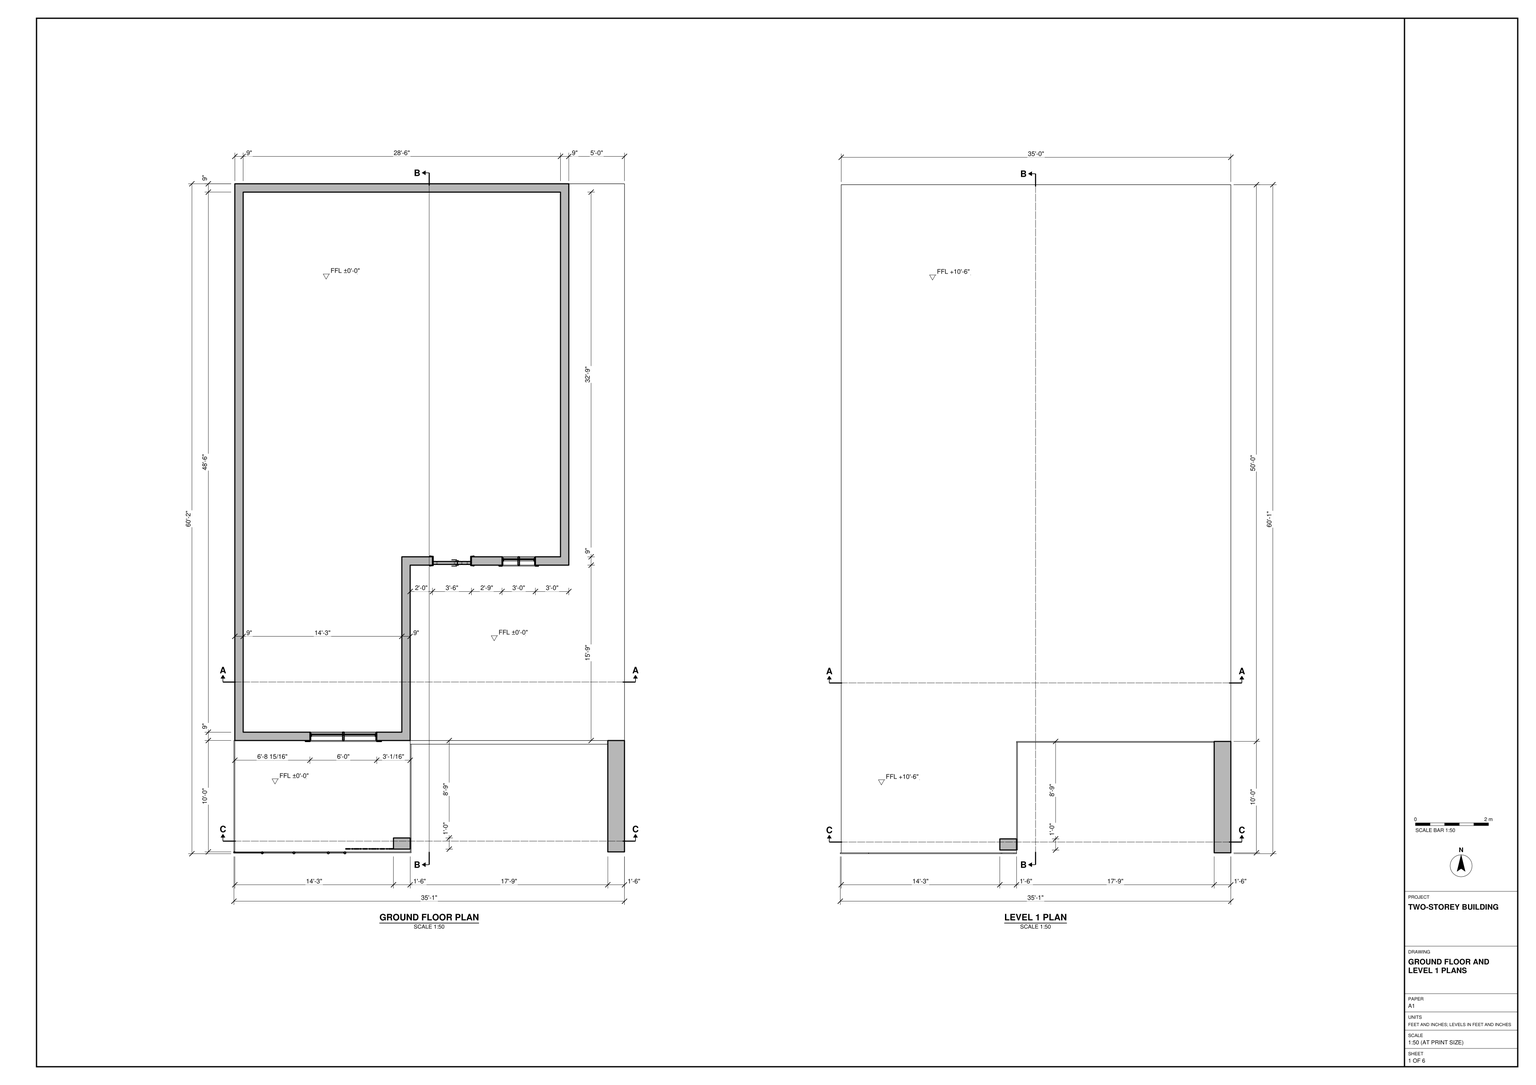
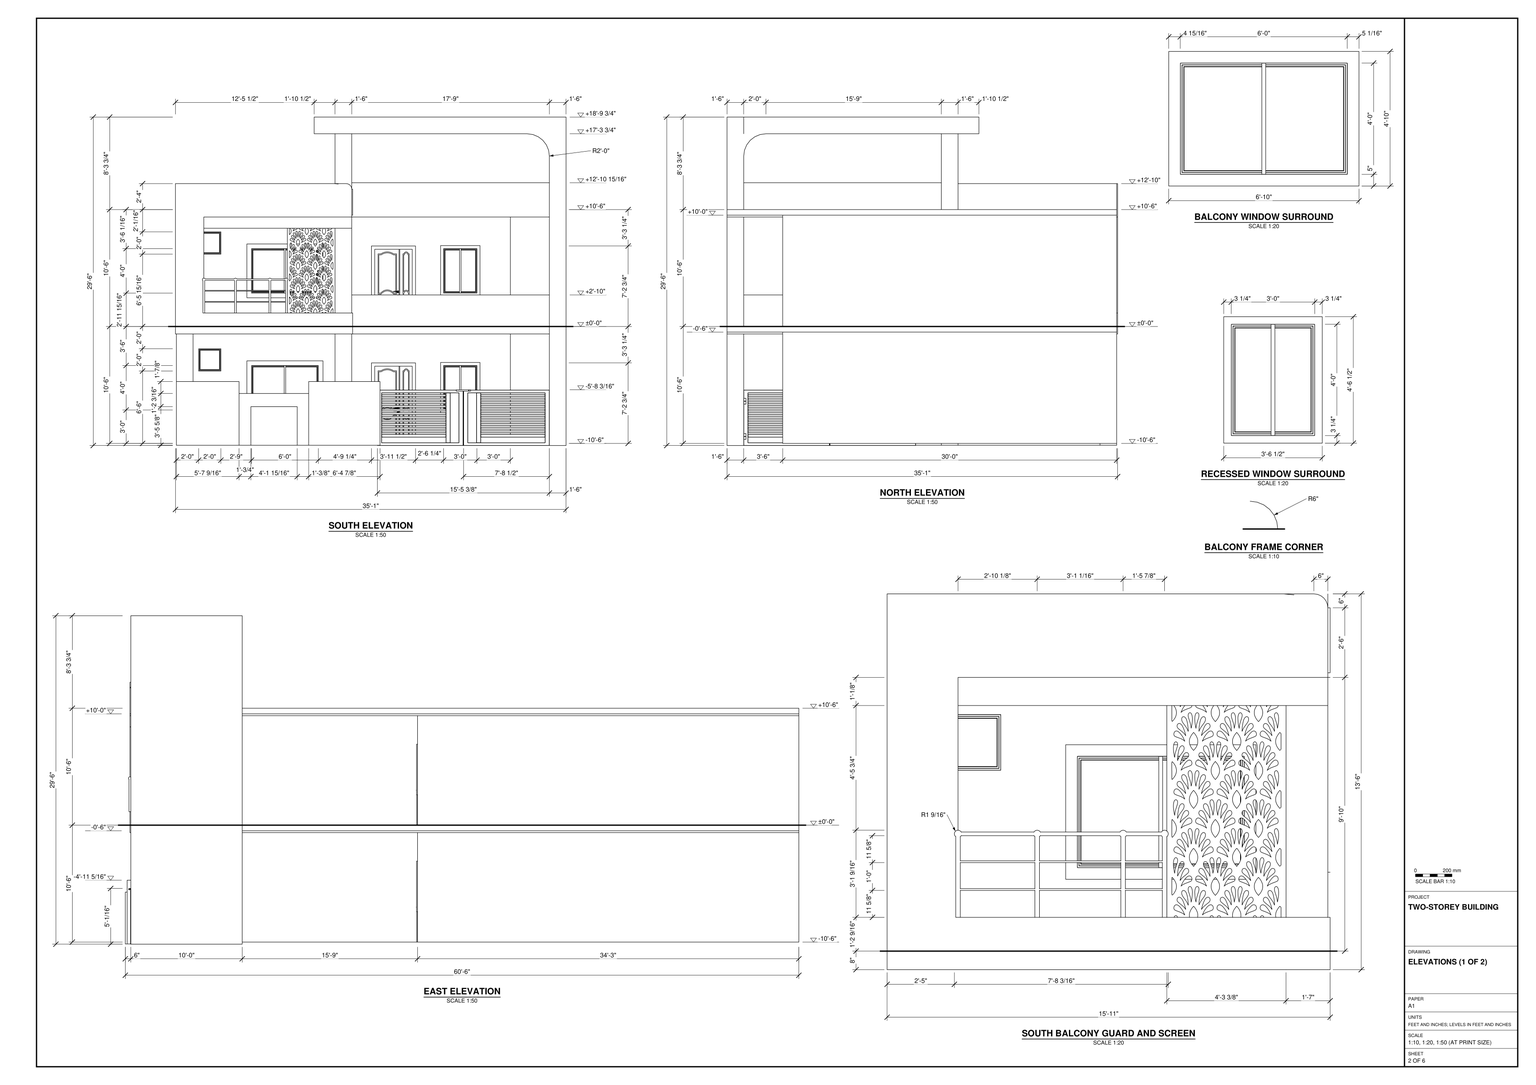
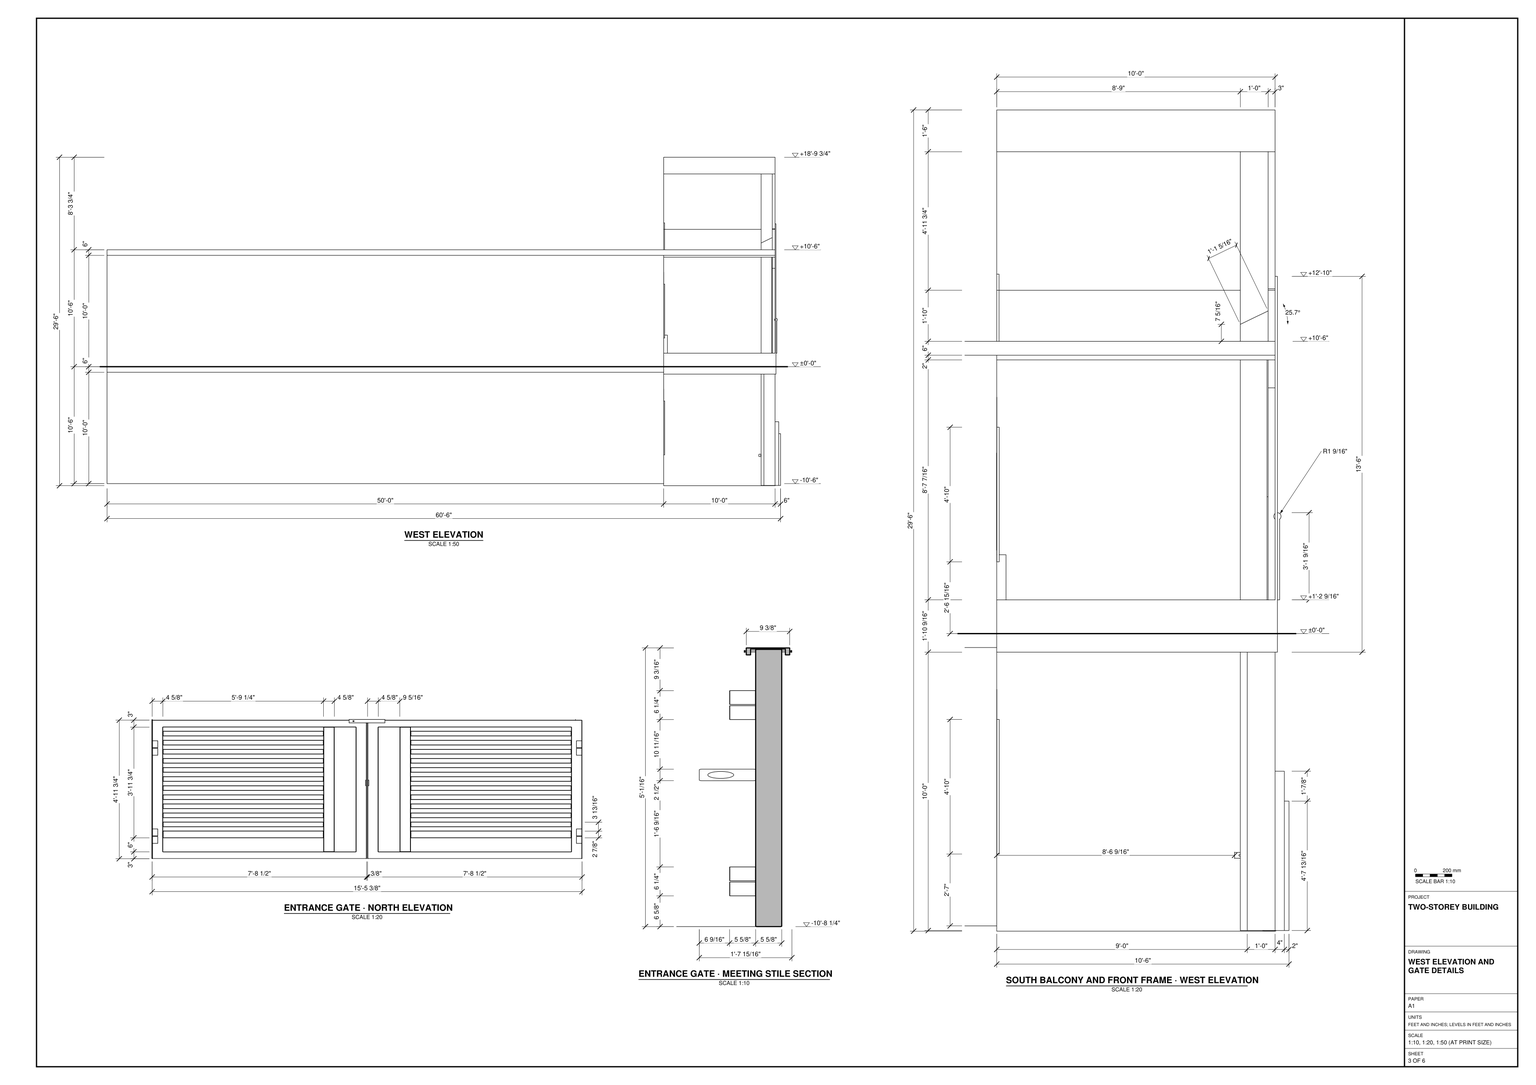
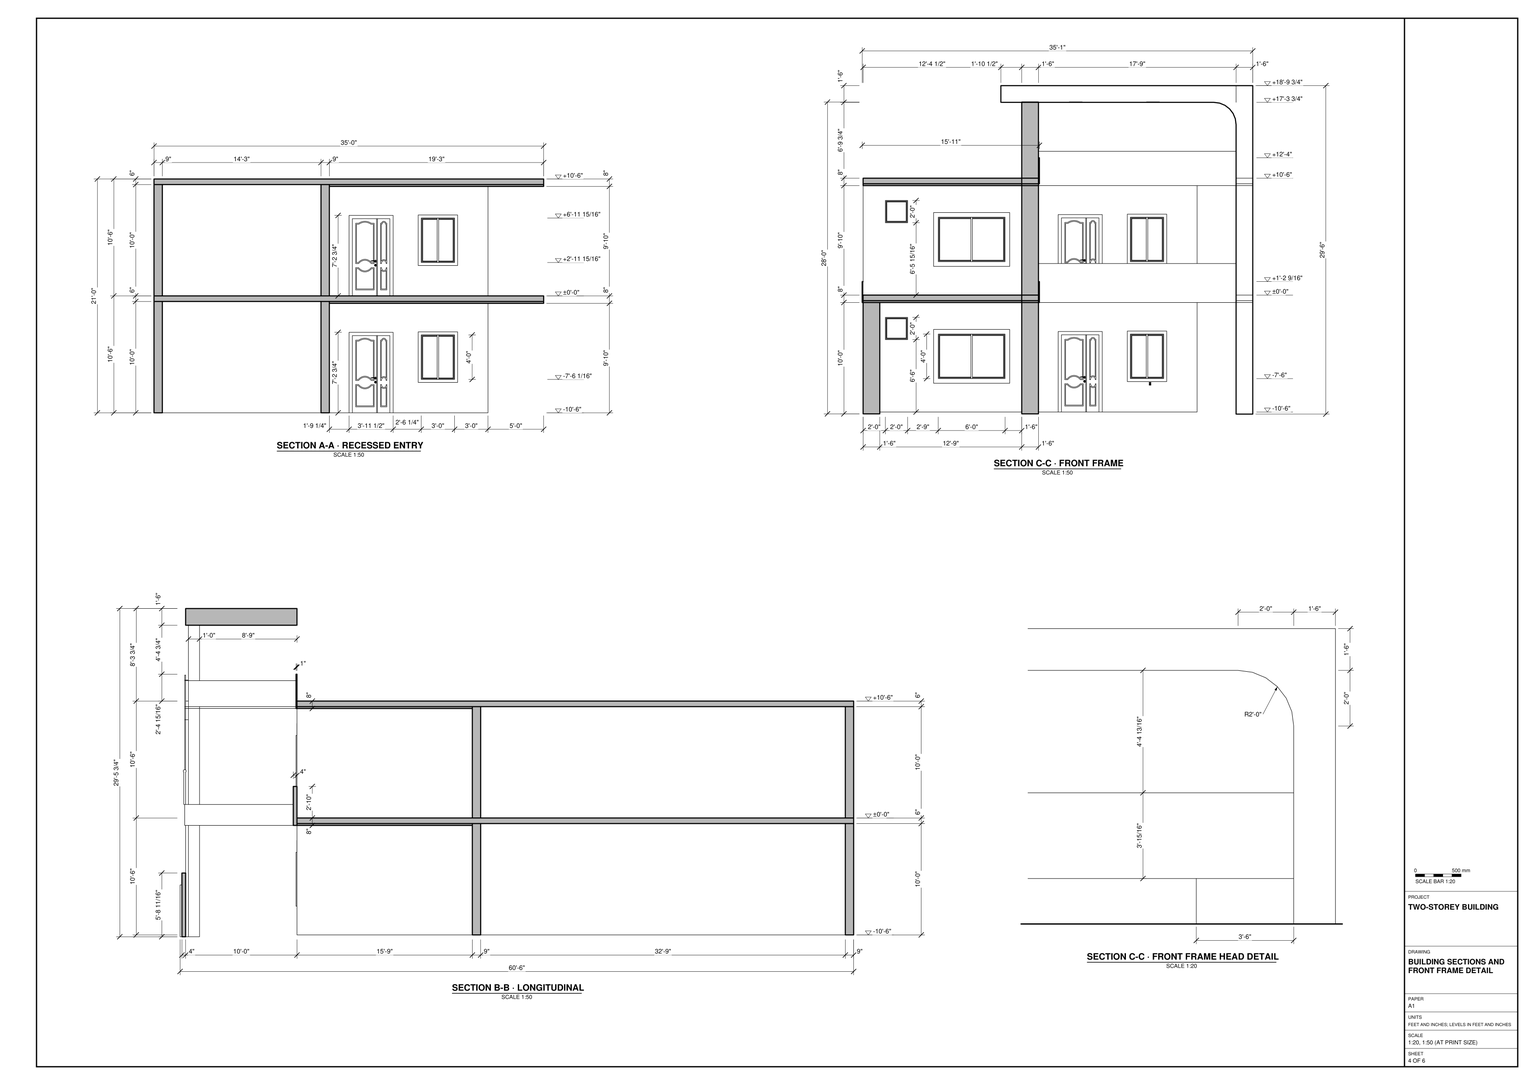
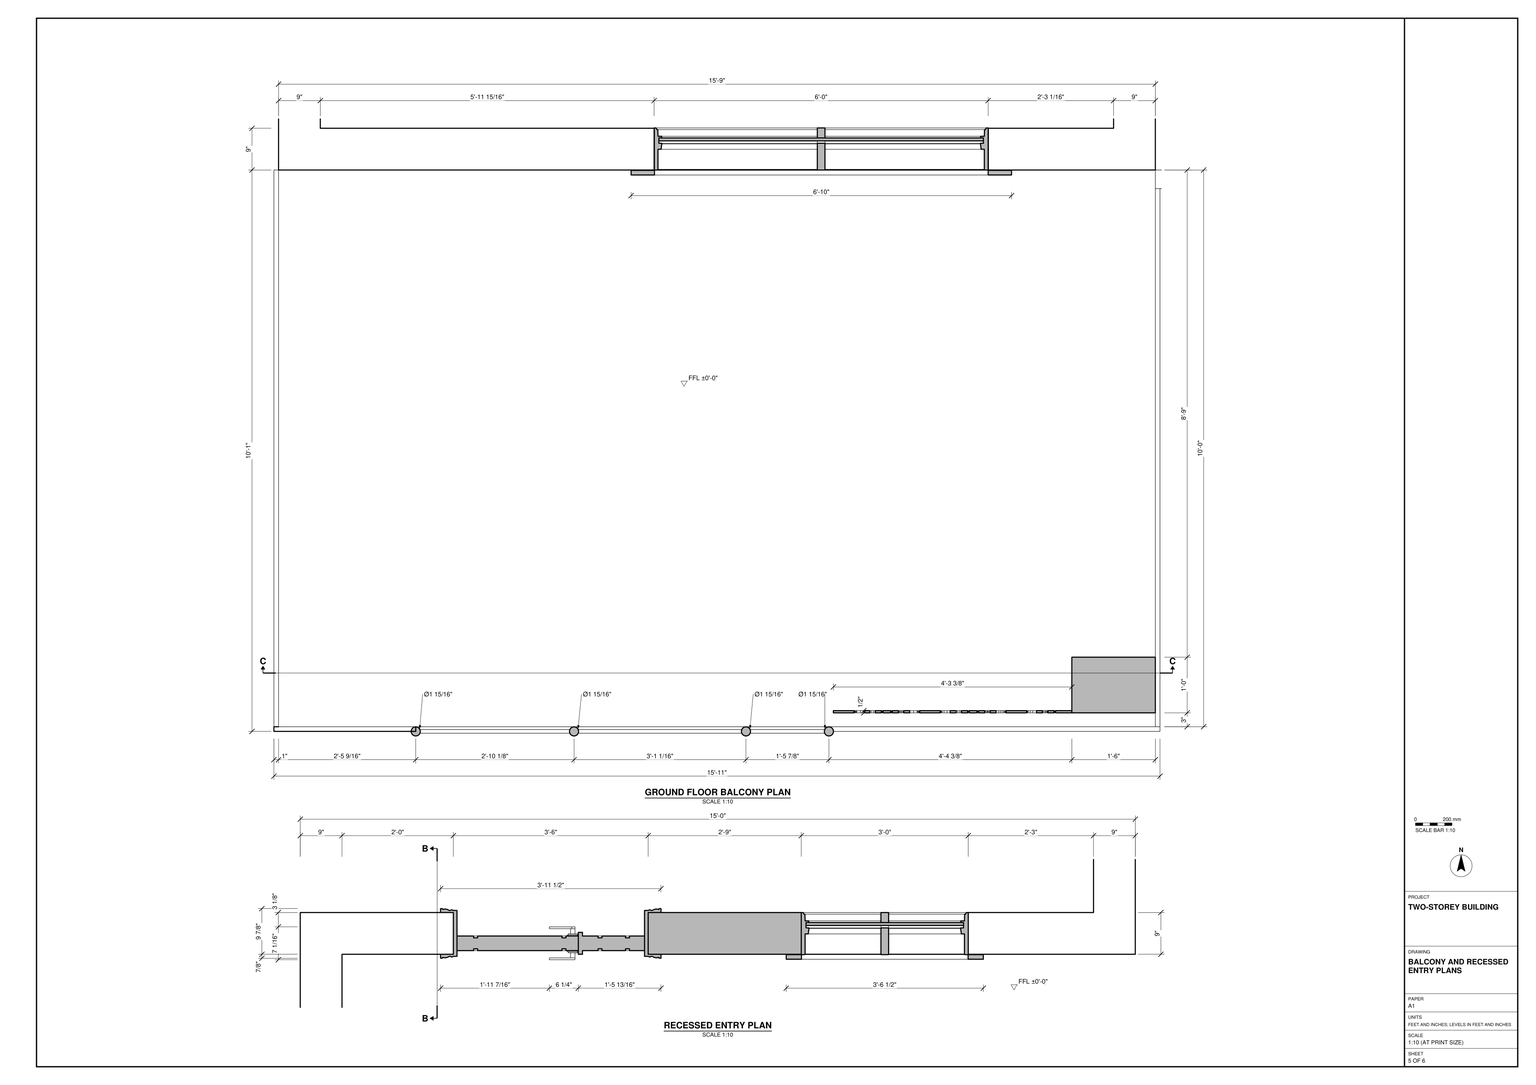
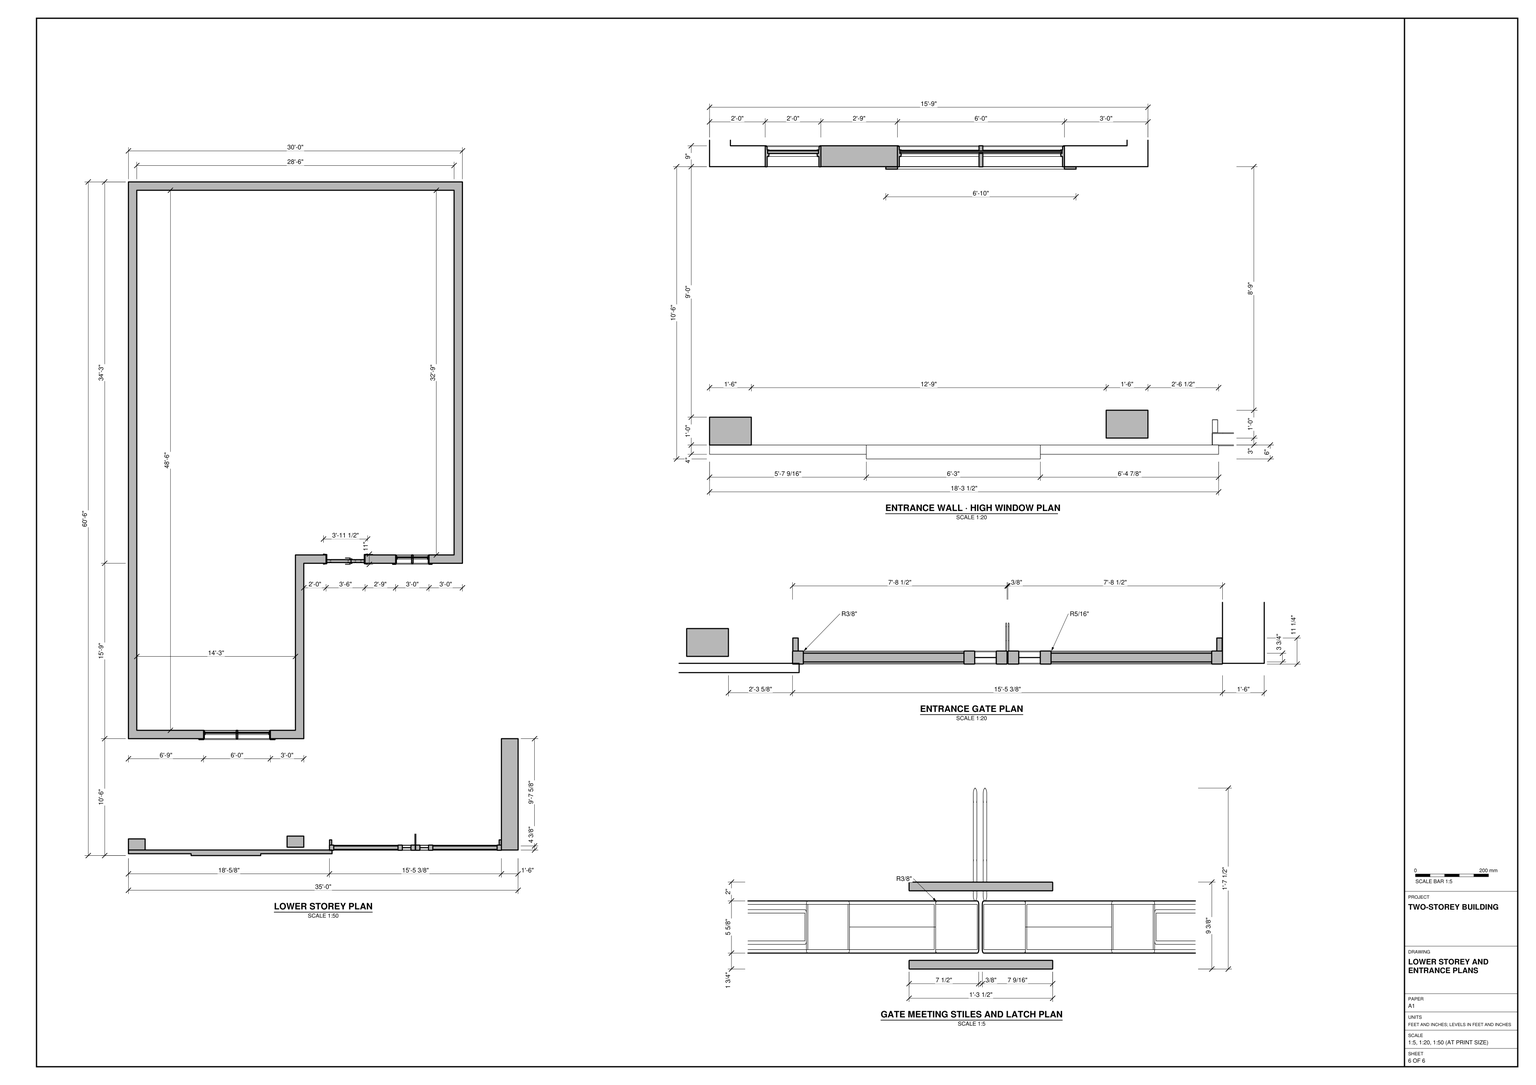
Build the two-storey building in SketchUp from task_files/diagram_01.pdf. Work in feet and inches. Set the overall width along X to 35'-1", the depth along Y to 60'-6", and the height to 29'-6". Use ±0'-0" for the ground floor and +10'-6" for Level 1.

Start with the ground-floor plan. Follow the 9" perimeter walls around the main enclosure, continuing the west wall forward and stepping the east portion back from the south entrance. Shape the floor slabs and flat roof to the outlines shown. Use the south elevation to locate the wider windows in the projecting bay and the doors and narrower windows in the recessed wall on both storeys. Include the window surrounds and divisions shown in the details.

Frame the south balcony with its horizontal guard and patterned screen. Distinguish the balcony frame from the taller overhead frame with its curved inside corner. At ground level, model the low frontage wall and the two-leaf slatted gate across the entrance.

Keep shell elements such as walls, slabs and roof, and each furniture or joinery piece shown, in separate groups or components. Use components for repeated parts. Decor and loose items may be any suitable library components. Save one SketchUp model as output_files/two_storey_building_with_its_balcony_and_entrance_gate.skp.

# SketchUp Ruby script. Lengths in inches.
U = 1.inch
M = Sketchup.active_model
def pt(a) = Geom::Point3d.new(a.map { |v| v * U })
def face(e, loops, mat)
  f = e.add_face(loops[0].map { |a| pt(a) })
  loops[1..].each { |l| e.add_face(l.map { |a| pt(a) }).erase! }
  f.material = f.back_material = mat if mat
  f
end
# faces: each face lists its corners as indices into pts; further lists are holes
def faces(e, pts, list, mat = nil) = list.each { |f| face(e, (f[0].is_a?(Array) ? f : [f]).map { |l| l.map { |i| pts[i] } }, mat) }
# xy, xz, yz: faces in a plane at the given z, y or x. An outline is a flat list of corners, or four numbers for a rectangle; further outlines are holes
def ring(l) = l.size == 4 ? [[l[0], l[1]], [l[2], l[1]], [l[2], l[3]], [l[0], l[3]]] : l.each_slice(2).to_a
def flat(e, list, mat, &to3) = list.each { |f| face(e, (f[0].is_a?(Array) ? f : [f]).map { |l| ring(l).map { |u, v| to3.(u, v) } }, mat) }
def xy(e, z, list, mat = nil) = flat(e, list, mat) { |x, y| [x, y, z] }
def xz(e, y, list, mat = nil) = flat(e, list, mat) { |x, z| [x, y, z] }
def yz(e, x, list, mat = nil) = flat(e, list, mat) { |y, z| [x, y, z] }
def lines(e, pts, list) = list.each { |a, b| e.add_line(pt(pts[a]), pt(pts[b])) }
# prism: a flat outline (further loops are holes) pulled along v
def prism(e, loops, v, mat = nil)
  f = face(e, loops, mat); d = Geom::Vector3d.new(v.map { |x| x * U })
  f.pushpull(f.normal.samedirection?(d) ? d.length : -d.length)
end
def box(e, o, s, mat = nil) = prism(e, [[o, [o[0] + s[0], o[1], o[2]], [o[0] + s[0], o[1] + s[1], o[2]], [o[0], o[1] + s[1], o[2]]]], [0, 0, s[2]], mat)
def at(x, y, z, deg = 0) = Geom::Transformation.translation(pt([x, y, z])) * Geom::Transformation.rotation(ORIGIN, Z_AXIS, deg.degrees)
def axes(o, x, y, z) = Geom::Transformation.new([*x, 0, *y, 0, *z, 0, *pt(o).to_a, 1])
def part(name) = M.definitions.add(name)
# library, detail: a bought-in or finely detailed component or shape, given as its bounding box
def library(name, o, s) = part(name).tap { |d| box(d.entities, o, s) }
def detail(e, o, s) = box(e.add_group.entities, o, s)
def put(e, d, t, mat = nil) = e.add_instance(d, t).tap { |i| i.material = mat if mat }
def group(e, t, mat = nil) = e.add_group.tap { |g| g.transformation = t; g.material = mat if mat }.entities
root = M.entities
M.materials.add("[Cladding Siding Tan]").color = [162, 126, 95]
M.materials.add("[Color B02]").color = [255, 178, 153]
M.materials.add("[Color B08]").color = [102, 25, 0]
M.materials.add("[Color C03]").color = [255, 178, 101]
M.materials.add("[Color D08]").color = [102, 76, 0]
M.materials.add("[Metal Silver]").color = [234, 233, 238]
M.materials.add("[Stone Marble]").color = [143, 138, 136]
M.materials.add("[Stone Vein Gray]").color = [166, 165, 165]
M.materials.add("[Translucent Glass Blue]").color = [100, 149, 237]
M.materials.add("[Wood Cherry Original]").color = [152, 86, 42]
M.materials.add("[Wood Veneer 01]").color = [120, 70, 37]
M.materials.add("[Wood Veneer 02]").color = [190, 128, 91]
c1 = library("Group\#19",[0,0,0],[1024,2048,10.625])
c2 = part("modren jali")
put(c2.entities,c1,axes([1490.25,379.44,-368.22],[1,0,0],[0,0,1],[0,-1,0]))
c3 = library("Main Gate",[0,-1.74,0],[119.75,5.32,60.06])
c4 = library("Group\#22",[0,0,0],[72,9.07,48])
c5 = library("Group\#3",[0,0,0],[47.51,11.03,86.76])
c6 = library("Group\#5",[0,0,0],[36,9.07,48])
c7 = part("Difference\#2")
xy(c7.entities,0,[[0,0,0,600,360,600,360,189,255,189,255,198,351,198,351,591,9,591,9,9,180,9,180,198,213,198,213,189,189,189,189,0]])
xy(c7.entities,36,[[81,0,153,9],[288,189,324,198]])
xy(c7.entities,78,[[24,0,48,9]])
xy(c7.entities,84,[[81,0,153,9],[213,189,255,198],[288,189,324,198]])
xy(c7.entities,102,[[24,0,48,9]])
xy(c7.entities,120,[[[0,0,189,0,189,189,360,189,360,600,0,600],[9,9,9,591,351,591,351,198,180,198,180,9]]])
xz(c7.entities,0,[[[0,0,189,120],[81,36,153,84],[24,78,48,102]]])
xz(c7.entities,9,[[[9,0,180,120],[81,36,153,84],[24,78,48,102]]])
xz(c7.entities,189,[[[189,0,213,0,213,84,255,84,255,0,360,0,360,120,189,120],[288,36,324,84]]])
xz(c7.entities,198,[[[180,0,180,120,351,120,351,0,255,0,255,84,213,84,213,0],[288,36,324,84]]])
xz(c7.entities,591,[[9,0,351,120]])
xz(c7.entities,600,[[0,0,360,120]])
yz(c7.entities,0,[[0,0,600,120]])
yz(c7.entities,9,[[9,0,591,120]])
yz(c7.entities,24,[[0,78,9,102]])
yz(c7.entities,48,[[0,78,9,102]])
yz(c7.entities,81,[[0,36,9,84]])
yz(c7.entities,153,[[0,36,9,84]])
yz(c7.entities,180,[[9,0,198,120]])
yz(c7.entities,189,[[0,0,189,120]])
yz(c7.entities,213,[[189,0,198,84]])
yz(c7.entities,255,[[189,0,198,84]])
yz(c7.entities,288,[[189,36,198,84]])
yz(c7.entities,324,[[189,36,198,84]])
yz(c7.entities,351,[[198,0,591,120]])
yz(c7.entities,360,[[189,0,600,120]])
c8 = part("Group15\#2")
box(c8.entities,[1.02,2.16,1.02],[21.96,1.15,21.96])
c9 = part("Group\#7")
put(c9.entities,c8,at(0,0,0),"[Translucent Glass Blue]")
g1 = group(c9.entities,at(0,0,0),"[Metal Silver]")
xy(g1,0,[[0,0,24,9]])
xy(g1,0.83,[[0.83,4.61,23.17,8.93]])
xy(g1,1.02,[[1.02,2.16,22.98,3.3125]])
xy(g1,1.61,[[1.61,1.8,22.39,2.16]])
xy(g1,1.65,[[1.65,3.3125,22.35,3.46]])
xy(g1,22.35,[[1.65,3.3125,22.35,3.46]])
xy(g1,22.39,[[1.61,1.8,22.39,2.16]])
xy(g1,22.98,[[1.02,2.16,22.98,3.3125]])
xy(g1,23.17,[[0.83,4.61,23.17,8.93]])
xy(g1,24,[[0,0,24,9]])
xz(g1,0,[[[0,0,24,24],[0.39,0.39,23.61,23.61]]])
xz(g1,0.36,[[[0.59,0.59,23.41,23.41],[0.79,0.79,23.21,23.21]]])
xz(g1,1.8,[[[0.83,0.83,23.17,23.17],[1.61,1.61,22.39,22.39]]])
xz(g1,2.16,[[[1.02,1.02,22.98,22.98],[1.61,1.61,22.39,22.39]]])
xz(g1,3.3125,[[[1.02,1.02,22.98,22.98],[1.65,1.65,22.35,22.35]]])
xz(g1,4.61,[[[0.83,0.83,23.17,23.17],[1.5,1.5,22.5,22.5]]])
xz(g1,9.07,[[[0.04,0.04,23.96,23.96],[0.75,0.75,23.25,23.25]]])
yz(g1,0,[[0,0,9,24]])
yz(g1,0.83,[[4.61,0.83,8.93,23.17]])
yz(g1,1.02,[[2.16,1.02,3.3125,22.98]])
yz(g1,1.61,[[1.8,1.61,2.16,22.39]])
yz(g1,1.65,[[3.3125,1.65,3.46,22.35]])
yz(g1,22.35,[[3.3125,1.65,3.46,22.35]])
yz(g1,22.39,[[1.8,1.61,2.16,22.39]])
yz(g1,22.98,[[2.16,1.02,3.3125,22.98]])
yz(g1,23.17,[[4.61,0.83,8.93,23.17]])
yz(g1,24,[[0,0,9,24]])
p = [[0,9,24],[0.04,9.07,23.96],[0.04,9.07,0.04],[0,9,0],[12,9.07,0.04],[23.96,9.07,0.04],
  [24,9,0],[12,9,0],[23.96,9.07,23.96],[24,9,24],[0.59,0.36,23.41],[0.39,0,23.61],
  [0.39,0,0.39],[0.59,0.36,0.59],[12,0,0.39],[23.61,0,0.39],[23.41,0.36,0.59],[12,0.36,0.59],
  [23.61,0,23.61],[23.41,0.36,23.41],[0.75,9.07,23.25],[0.83,8.93,23.17],[0.83,8.93,0.83],[0.75,9.07,0.75],
  [12,8.93,0.83],[23.17,8.93,0.83],[23.25,9.07,0.75],[12,9.07,0.75],[23.17,8.93,23.17],[23.25,9.07,23.25],
  [0.83,1.8,23.17],[0.79,0.36,23.21],[0.79,0.36,0.79],[0.83,1.8,0.83],[12,0.36,0.79],[23.21,0.36,0.79],
  [23.17,1.8,0.83],[12,1.8,0.83],[23.21,0.36,23.21],[23.17,1.8,23.17],[1.5,4.61,22.5],[1.65,3.46,22.35],
  [1.65,3.46,1.65],[1.5,4.61,1.5],[12,3.46,1.65],[22.35,3.46,1.65],[22.5,4.61,1.5],[12,4.61,1.5],
  [22.35,3.46,22.35],[22.5,4.61,22.5]]
faces(g1,p,[[0,1,2,3],[4,5,6,7,3,2],[6,5,8,9],[10,11,12,13],[14,15,16,17,13,12],[16,15,18,19],[20,21,22,23],[24,25,26,27,23,22],
  [26,25,28,29],[30,31,32,33],[34,35,36,37,33,32],[36,35,38,39],[40,41,42,43],[44,45,46,47,43,42],[46,45,48,49],[49,48,41,40],
  [39,38,31,30],[29,28,21,20],[19,18,11,10],[9,8,1,0]])
c10 = library("Group\#2",[0,0,0],[72,9.07,48])
c11 = part("Group\#9")
prism(c11.entities,[[[82.01,1,58.01],[82.01,1,0],[0,1,0],[0,1,58.01]],[[5.04,1,52.97],[5.04,1,5.04],[76.97,1,5.04],[76.97,1,52.97]]],[0,-1,0])
c12 = part("Group\#10")
prism(c12.entities,[[[42.49,0,54.49],[0,0,54.49],[0,0,0],[42.49,0,0]],[[3.28,0,51.21],[39.21,0,51.21],[39.21,0,3.28],[3.28,0,3.28]]],[0,1,0])
c13 = library("Group\#23",[0,0,0],[36,9.07,48])
c14 = library("Group\#12",[0,0,0],[231,600,2])
c15 = library("Group\#13",[0,0,0],[231,600,2])
c16 = library("Group\#14",[0,0,0],[189,120,2])
c17 = library("Group\#21",[0,0,0],[189,120,2])
c18 = part("Difference\#1")
xy(c18.entities,0,[[0,0,0,600,360,600,360,189,255,189,255,198,351,198,351,591,9,591,9,9,180,9,180,198,213,198,213,189,189,189,189,0]])
xy(c18.entities,36,[[81,0,153,9],[288,189,324,198]])
xy(c18.entities,78,[[24,0,48,9]])
xy(c18.entities,84,[[81,0,153,9],[213,189,255,198],[288,189,324,198]])
xy(c18.entities,102,[[24,0,48,9]])
xy(c18.entities,120,[[[0,0,189,0,189,189,360,189,360,600,0,600],[9,9,9,591,351,591,351,198,180,198,180,9]]])
xz(c18.entities,0,[[[0,0,189,120],[81,36,153,84],[24,78,48,102]]],"[Cladding Siding Tan]")
xz(c18.entities,9,[[[9,0,180,120],[81,36,153,84],[24,78,48,102]]])
xz(c18.entities,189,[[[189,0,213,0,213,84,255,84,255,0,360,0,360,120,189,120],[288,36,324,84]]])
xz(c18.entities,198,[[[180,0,180,120,351,120,351,0,255,0,255,84,213,84,213,0],[288,36,324,84]]])
xz(c18.entities,591,[[9,0,351,120]])
xz(c18.entities,600,[[0,0,360,120]])
yz(c18.entities,0,[[0,0,600,120]])
yz(c18.entities,9,[[9,0,591,120]])
yz(c18.entities,24,[[0,78,9,102]])
yz(c18.entities,48,[[0,78,9,102]])
yz(c18.entities,81,[[0,36,9,84]])
yz(c18.entities,153,[[0,36,9,84]])
yz(c18.entities,180,[[9,0,198,120]])
yz(c18.entities,189,[[0,0,189,120]])
yz(c18.entities,213,[[189,0,198,84]])
yz(c18.entities,255,[[189,0,198,84]])
yz(c18.entities,288,[[189,36,198,84]])
yz(c18.entities,324,[[189,36,198,84]])
yz(c18.entities,351,[[198,0,591,120]])
yz(c18.entities,360,[[189,0,600,120]])
c19 = library("Group\#38",[0,0,0],[92.21,3.15,37.57])
prism(root,[[[232.19,63.35,333.73],[233.86,62.6,333.73],[235.28,61.44,333.73],[236.35,59.96,333.73],[237,58.25,333.73],[237.18,56.43,333.73],[236.89,54.63,333.73],[236.14,52.96,333.73],[234.98,51.55,333.73],[233.5,50.48,333.73],[231.79,49.83,333.73],[229.98,49.64,333.73],[228.17,49.9375,333.73],[226.51,50.68,333.73],[225.09,51.84,333.73],[224.02,53.32,333.73],[223.37,55.03,333.73],[223.1875,56.85,333.73],[223.48,58.65,333.73],[224.23,60.32,333.73],[225.38,61.73,333.73],[226.86,62.8,333.73],[228.57,63.45,333.73],[230.39,63.64,333.73]]],[0,0,0.5])
prism(root,[[[315.44,63.35,333.73],[317.11,62.6,333.73],[318.53,61.44,333.73],[319.6,59.96,333.73],[320.25,58.25,333.73],[320.43,56.43,333.73],[320.14,54.63,333.73],[319.39,52.96,333.73],[318.23,51.55,333.73],[316.75,50.48,333.73],[315.04,49.83,333.73],[313.23,49.64,333.73],[311.42,49.9375,333.73],[309.76,50.68,333.73],[308.34,51.84,333.73],[307.27,53.32,333.73],[306.62,55.03,333.73],[306.4375,56.85,333.73],[306.73,58.65,333.73],[307.48,60.32,333.73],[308.63,61.73,333.73],[310.11,62.8,333.73],[311.82,63.45,333.73],[313.64,63.64,333.73]]],[0,0,0.5])
xy(root,231.87,[[30.57,5,190,6]])
xy(root,244,[[30.57,5,190,6],[190,125,403,126]])
xy(root,246,[[190,9,191,125]])
xy(root,274,[[190,9,191,125]])
xy(root,280.96,[[190,125,403,126]])
xz(root,5,[[30.57,231.87,190,244]],"[Wood Veneer 01]")
xz(root,6,[[30.57,231.87,190,244]])
xz(root,9,[[190,246,191,274]])
xz(root,125,[[190,244,403,244,403,280.96,190,280.96,190,274,191,274,191,246,190,246]],"[Stone Vein Gray]")
xz(root,126,[[190,244,403,280.96]])
yz(root,30.57,[[5,231.87,6,244]])
yz(root,190,[[5,231.87,6,231.95],[5,231.95,6,244],[6,231.95,9,244],[5,244,9,246],[125,244,126,246],
  [5,246,9,274],[5,274,9,274.64],[125,274,126,280.96]])
yz(root,191,[[9,246,125,274]])
yz(root,403,[[125,244,126,280.96]])
# 1 loose lines left out
put(root,c2,axes([246.81,26.01,147.22],[-0.0502,0,0],[0,-0.04483,0],[0,0,0.05762]))
put(root,c3,axes([217.65,16.93,-2.27],[1.54782,0,0],[0,-3.7464,0],[0,0,1]))
put(root,c4,at(154,135,36,180))
put(root,c5,at(211.24,313.82,0))
put(root,c6,at(325,324,161.96,180))
put(root,c7,at(1,126,0),"[Color B02]")
put(root,c9,at(49,135,78,180))
put(root,c5,at(211.24,313.82,126))
put(root,c10,at(153.96,135.07,161.96,180),"[Color B08]")
put(root,c11,at(77,124.93,31))
put(root,c12,at(285.76,313.93,32.76))
put(root,c12,at(285.76,313.93,158.72))
put(root,c13,at(325,324,35.96,180),"[Color B08]")
put(root,c9,at(49,135,203.96,180))
g2 = group(root,at(1,126,246))
prism(g2,[[[0,-120,0],[0,600,0],[420,600,0],[420,0,0],[189,0,0],[189,-120,0]]],[0,0,6])
put(root,c14,at(190,126,244),"[Wood Veneer 02]")
put(root,c15,at(190,126,118),"[Wood Veneer 02]")
put(root,c16,at(1,6,244),"[Wood Veneer 02]")
g3 = group(root,at(1,6,-2))
box(g3,[0,0,0],[18,12,120])
g4 = group(root,at(403,6,-2.27))
xy(g4,0,[[0,0,18,120]])
xy(g4,336,[[-253.5,0,-24,120]])
xy(g4,354,[[-253.5,0,18,120]])
xz(g4,0,[[0,0,18,0,18,354,-253.5,354,-253.5,336,0,336],[0,312,0,336,-24,336,-17.79,335.18,-12,332.78,-7.03,328.97,-3.22,324,-0.82,318.21]])
xz(g4,120,[[0,0,18,354],[0,312,-0.82,318.21,-3.22,324,-7.03,328.97,-12,332.78,-17.79,335.18,-24,336,0,336],[-253.5,336,0,354]])
yz(g4,-253.5,[[0,336,120,354]])
yz(g4,0,[[0,0,120,312]])
yz(g4,18,[[0,0,120,354]])
p = [[0,120,312],[0,0,312],[-0.82,0,318.21],[-0.82,120,318.21],[-3.22,0,324],[-3.22,120,324],
  [-7.03,0,328.97],[-7.03,120,328.97],[-12,0,332.78],[-12,120,332.78],[-17.79,0,335.18],[-17.79,120,335.18],
  [-24,0,336],[-24,120,336]]
faces(g4,p,[[0,1,2,3],[3,2,4,5],[5,4,6,7],[7,6,8,9],[9,8,10,11],[11,10,12,13]])
put(root,c17,at(1,6,118),"[Wood Veneer 02]")
g5 = group(root,at(172,9,-2))
xy(g5,0,[[0,0,18,12]])
xy(g5,336,[[0,0,18,12]])
xz(g5,0,[[0,0,18,267.1]])
xz(g5,0,[[0,267.1,18,336]],"[Stone Marble]")
xz(g5,12,[[0,0,18,336]])
yz(g5,0,[[0,0,0,267.1,12,261.32,12,0],[12,261.32,0,267.1,0,336,12,336]])
yz(g5,18,[[0,0,12,0,12,261.32,0,267.1]])
yz(g5,18,[[12,261.32,12,336,0,336,0,267.1]],"[Stone Vein Gray]")
# 1 loose lines left out
g6 = group(root,at(1,126,120))
prism(g6,[[[0,-120,0],[0,600,0],[420,600,0],[420,0,0],[189,0,0],[189,-120,0]]],[0,0,6])
g7 = group(root,at(190,122,118),"[Stone Vein Gray]")
box(g7,[0,0,0],[213,4,42])
put(root,c18,at(1,126,126),"[Color B02]")
put(root,c11,at(77,124.93,156.96))
g8 = group(root,at(0,5,118),"[Wood Cherry Original]")
xy(g8,0,[[0,0,191,1],[0,1,1,121],[190,1,191,117]])
xy(g8,22.55,[[30.57,0,191,1],[0,1,1,121],[190,1,191,117]])
xy(g8,126,[[30.57,0,190,1]])
xy(g8,162,[[0,0,30.57,1],[30.57,0,184,1]])
xz(g8,0,[[0,0,191,0,191,22.55,30.57,22.55,30.57,126,190,126,190,156,189.8,157.55,189.2,159,188.24,160.24,187,161.2,185.55,161.8,184,162,0,162]])
xz(g8,1,[[0,22.55,1,126],[0,126,1,162]])
xz(g8,117,[[190,0,191,22.55]])
xz(g8,121,[[0,0,1,22.55]])
yz(g8,0,[[0,0,0,162,1,162,1,22.55,121,22.55,121,0]])
yz(g8,30.57,[[0,22.55,1,126]])
yz(g8,190,[[0,126,1,156]])
yz(g8,191,[[0,0,117,22.55]])
p = [[189.8,1,157.55],[189.8,0,157.55],[190,0,156],[190,1,156],[189.2,1,159],[189.2,0,159],
  [188.24,1,160.24],[188.24,0,160.24],[187,1,161.2],[187,0,161.2],[185.55,1,161.8],[185.55,0,161.8],
  [184,1,162],[184,0,162]]
faces(g8,p,[[0,1,2,3],[4,5,1,0],[6,7,5,4],[8,9,7,6],[10,11,9,8],[12,13,11,10]])
g9 = group(root,at(1,0,-2))
xy(g9,0,[[67.58,0,67.58,2,0,2,0,6,219.47,6,219.47,2,142.6,2,142.6,0,130.24,0,130.24,2,80.31,2,80.31,0]])
xy(g9,41.625,[[80.31,0,130.24,2]])
xy(g9,55.8,[[67.58,0,142.6,6]])
xy(g9,68.68,[[0,2,67.58,6],[142.6,2,219.47,6]])
xz(g9,0,[[67.58,0,80.31,0,80.31,41.625,130.24,41.625,130.24,0,142.6,0,142.6,55.8,67.58,55.8]])
xz(g9,2,[[80.31,0,130.24,41.625]],"[Color C03]")
xz(g9,2,[[0,0,67.58,68.68],[142.6,0,219.47,68.68]],"[Color D08]")
xz(g9,6,[[0,0,0,68.68,67.58,68.68,67.58,55.8,142.6,55.8,142.6,68.68,219.47,68.68,219.47,0]])
yz(g9,0,[[2,0,6,68.68]])
yz(g9,67.58,[[0,0,2,55.8],[2,55.8,6,68.68]])
yz(g9,80.31,[[0,0,2,41.625]])
yz(g9,130.24,[[0,0,2,41.625]])
yz(g9,142.6,[[0,0,2,55.8],[2,55.8,6,68.68]])
yz(g9,219.47,[[2,0,6,68.68]])
put(root,c19,at(28.99,3.43,140.55))
